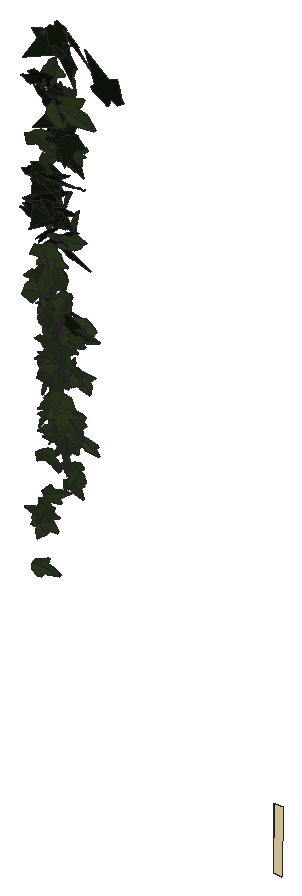
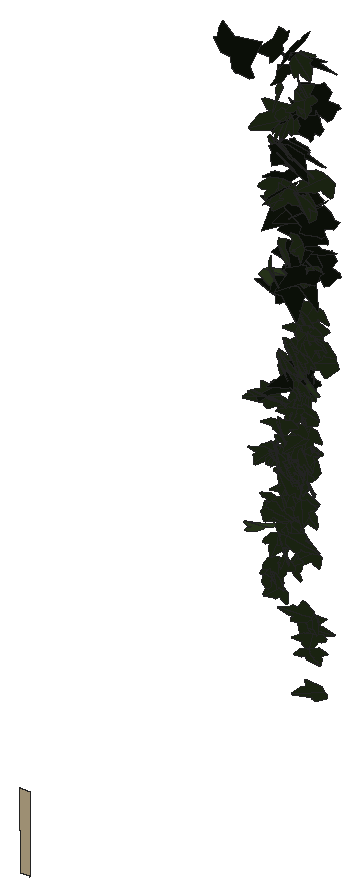
# SketchUp Ruby script. Lengths in inches.
U = 1.inch
M = Sketchup.active_model
def pt(a) = Geom::Point3d.new(a.map { |v| v * U })
def face(e, loops, mat)
  f = e.add_face(loops[0].map { |a| pt(a) })
  loops[1..].each { |l| e.add_face(l.map { |a| pt(a) }).erase! }
  f.material = f.back_material = mat if mat
  f
end
# faces: each face lists its corners as indices into pts; further lists are holes
def faces(e, pts, list, mat = nil) = list.each { |f| face(e, (f[0].is_a?(Array) ? f : [f]).map { |l| l.map { |i| pts[i] } }, mat) }
# xy, xz, yz: faces in a plane at the given z, y or x. An outline is a flat list of corners, or four numbers for a rectangle; further outlines are holes
def ring(l) = l.size == 4 ? [[l[0], l[1]], [l[2], l[1]], [l[2], l[3]], [l[0], l[3]]] : l.each_slice(2).to_a
def flat(e, list, mat, &to3) = list.each { |f| face(e, (f[0].is_a?(Array) ? f : [f]).map { |l| ring(l).map { |u, v| to3.(u, v) } }, mat) }
def xy(e, z, list, mat = nil) = flat(e, list, mat) { |x, y| [x, y, z] }
def xz(e, y, list, mat = nil) = flat(e, list, mat) { |x, z| [x, y, z] }
def yz(e, x, list, mat = nil) = flat(e, list, mat) { |y, z| [x, y, z] }
def lines(e, pts, list) = list.each { |a, b| e.add_line(pt(pts[a]), pt(pts[b])) }
# prism: a flat outline (further loops are holes) pulled along v
def prism(e, loops, v, mat = nil)
  f = face(e, loops, mat); d = Geom::Vector3d.new(v.map { |x| x * U })
  f.pushpull(f.normal.samedirection?(d) ? d.length : -d.length)
end
def box(e, o, s, mat = nil) = prism(e, [[o, [o[0] + s[0], o[1], o[2]], [o[0] + s[0], o[1] + s[1], o[2]], [o[0], o[1] + s[1], o[2]]]], [0, 0, s[2]], mat)
def at(x, y, z, deg = 0) = Geom::Transformation.translation(pt([x, y, z])) * Geom::Transformation.rotation(ORIGIN, Z_AXIS, deg.degrees)
def axes(o, x, y, z) = Geom::Transformation.new([*x, 0, *y, 0, *z, 0, *pt(o).to_a, 1])
def part(name) = M.definitions.add(name)
# library, detail: a bought-in or finely detailed component or shape, given as its bounding box
def library(name, o, s) = part(name).tap { |d| box(d.entities, o, s) }
def detail(e, o, s) = box(e.add_group.entities, o, s)
def put(e, d, t, mat = nil) = e.add_instance(d, t).tap { |i| i.material = mat if mat }
def group(e, t, mat = nil) = e.add_group.tap { |g| g.transformation = t; g.material = mat if mat }.entities
root = M.entities
M.materials.add("1026 AP 7946 SUNNY SIDE UP").color = [254, 231, 186]
M.materials.add("efeu1").color = [18, 25, 13]
M.materials.add("efeu2").color = [43, 57, 29]
c1 = part("ivyleaf_10")
p = [[0,0.5,-0.03],[-0.0625,2.02,-0.43],[-0.19,2.01,-0.46],[-0.54,1.05,-0.29],[-0.52,0.625,-0.18],[-0.83,0.76,-0.28],
  [-1.16,0.64,-0.33],[-1.15,0.33,-0.24],[-0.77,-0.39,0.02],[-0.3,-0.51,0.16],[0.04,-0.48,0.23],[-0.02,2.01,-0.4375],
  [-0.06,2.01,-0.43],[0.04,-0.49,0.23],[0.67,-0.49,0.14],[1.38,0.36,-0.2],[1.375,0.51,-0.24],[0.81,0.65,-0.19],
  [0.62,0.59,-0.15],[0.6,1.09,-0.28],[0.5,1.23,-0.31]]
faces(c1.entities,p,[[0,1,2,3,4,5,6,7,8,9,10],[11,12,0,13,14,15,16,17,18,19,20]],"efeu2")
c2 = part("ivyleaf_9")
p = [[1.54,2.16,1.25],[1.36,2.04,1.19],[-0.21,0.99,0.68],[-0.71,1.11,0.82],[-0.85,0.86,0.67],[-0.8,0.17,0.21],
  [-0.9,-0.01,0.1],[-0.67,-0.16,-0.02],[-0.08,-0.08,-0.05],[-0.03,-0.6,-0.4],[0.65,-0.88,-0.66],[0.83,-0.6,-0.49],
  [1.29,-0.42,-0.43],[1.8125,-0.07,-0.26],[1.21,0.44,0.15]]
faces(c2.entities,p,[[0,1,2,3,4,5,6,7,8,9,10,11,12,13,14]],"efeu1")
xz(root,213.099,[[153.231,245.999,153.241,247.999,152.988,248,152.981,246]],"1026 AP 7946 SUNNY SIDE UP")
p = [[152.981,213.099,246],[152.988,213.099,248],[152.981,213.1,248],[152.978,213.099,246]]
faces(root,p,[[0,1,2,3]],"1026 AP 7946 SUNNY SIDE UP")
put(root,c1,axes([145.59,212.75,264.89],[-0.28973,-0.04705,-0.17397],[0.26689,0.0118,-0.19442],[0.06726,-0.24948,0.0221]),"1026 AP 7946 SUNNY SIDE UP")
put(root,c2,axes([145.47,212.61,262.8],[0.36964,-0.02084,0.11456],[0.16957,-0.03713,-0.242],[0.05438,0.25744,-0.02409]),"1026 AP 7946 SUNNY SIDE UP")
put(root,c1,axes([146.01,212.67,254.15],[0.01993,-0.00468,-0.21341],[-0.32565,0.00536,-0.01315],[0.00886,0.20745,-0.00326]),"1026 AP 7946 SUNNY SIDE UP")
put(root,c1,axes([145.77,212.74,260.93],[-0.36692,-0.08893,-0.03495],[0.07197,-0.02757,-0.25381],[0.1309,-0.23411,0.04158]),"1026 AP 7946 SUNNY SIDE UP")
put(root,c1,axes([145.84,212.76,260.0625],[-0.22002,0.18793,0.06334],[-0.10512,0.02457,-0.23808],[-0.29205,-0.15042,0.03797]),"1026 AP 7946 SUNNY SIDE UP")
put(root,c1,axes([145.82,213.1875,267.8],[-0.05734,-0.22404,0.10374],[-0.00507,-0.10264,-0.23411],[0.38702,-0.03454,0.0123]),"1026 AP 7946 SUNNY SIDE UP")
put(root,c1,axes([145.82,212.67,261.2],[-0.02168,-0.25461,-0.00797],[-0.00088,0.00633,-0.26264],[0.40047,-0.01377,-0.00101]),"1026 AP 7946 SUNNY SIDE UP")
put(root,c1,axes([145.54,212.5625,260.49],[-0.05462,-0.05264,-0.23677],[0.34552,0.07617,-0.05181],[0.13313,-0.21929,0.03733]),"1026 AP 7946 SUNNY SIDE UP")
put(root,c1,axes([145.8,212.92,258.95],[-0.32874,0.02394,-0.0091],[0.01137,-0.01548,-0.21636],[-0.03855,-0.20869,0.01377]),"1026 AP 7946 SUNNY SIDE UP")
put(root,c1,axes([145.55,213.07,259.4375],[0.00437,-0.01694,-0.21177],[0.28532,-0.09735,0.01023],[-0.15389,-0.18097,0.01295]),"1026 AP 7946 SUNNY SIDE UP")
put(root,c1,axes([145.84,212.98,258.43],[-0.04466,-0.19756,0.04918],[-0.01328,-0.04815,-0.20589],[0.31972,-0.02959,-0.00168]),"1026 AP 7946 SUNNY SIDE UP")
put(root,c1,axes([145.8,212.84,253.71],[0.27005,0.08927,-0.06744],[-0.07271,-0.05294,-0.19813],[-0.15866,0.17619,-0.02398]),"1026 AP 7946 SUNNY SIDE UP")
put(root,c1,axes([145.77,212.99,257.84],[0.21885,-0.15832,0.05318],[0.03274,-0.05137,-0.2167],[0.26024,0.13961,-0.01746]),"1026 AP 7946 SUNNY SIDE UP")
put(root,c1,axes([145.8125,213.09,257.24],[-0.06075,-0.20631,-0.01788],[0.03651,0.01204,-0.21512],[0.32334,-0.04012,0.02093]),"1026 AP 7946 SUNNY SIDE UP")
put(root,c1,axes([145.82,213.05,257.68],[-0.18649,0.16259,0.04429],[0.05147,-0.02813,0.20693],[0.25901,0.12266,-0.00924]),"1026 AP 7946 SUNNY SIDE UP")
put(root,c1,axes([146.04,213.08,256.36],[-0.10447,-0.0008,0.20049],[-0.27494,-0.09005,-0.0624],[0.13437,-0.18488,0.02819]),"1026 AP 7946 SUNNY SIDE UP")
put(root,c1,axes([145.79,213.24,261.26],[-0.03188,0.03985,-0.2062],[-0.02068,-0.20121,-0.04103],[-0.32059,0.00902,0.02315]),"1026 AP 7946 SUNNY SIDE UP")
put(root,c1,axes([145.85,212.97,258.5],[-0.1948,-0.16449,0.00997],[0.00967,-0.01788,-0.21163],[0.259,-0.12305,0.0154]),"1026 AP 7946 SUNNY SIDE UP")
put(root,c2,axes([145.58,212.58,266.6875],[0.37695,0.05787,0.09665],[0.15159,-0.00285,-0.2529],[-0.0831,0.2573,-0.02295]),"1026 AP 7946 SUNNY SIDE UP")
put(root,c1,axes([145.67,212.86,259.91],[0.1097,-0.17416,-0.087],[0.14964,-0.04622,0.18104],[-0.26425,-0.09847,0.0664]),"1026 AP 7946 SUNNY SIDE UP")
put(root,c1,axes([145.77,212.87,257.9],[-0.09767,-0.16191,0.13668],[0.05553,0.12927,0.17907],[-0.32536,0.07067,-0.01047]),"1026 AP 7946 SUNNY SIDE UP")
put(root,c1,axes([145.82,213.02,266.74],[0.15259,0.21371,-0.05953],[-0.02659,-0.05708,-0.24199],[-0.34759,0.09819,-0.00762]),"1026 AP 7946 SUNNY SIDE UP")
put(root,c1,axes([145.91,212.84,256.95],[-0.01576,-0.18278,0.09988],[-0.008,-0.09786,-0.18915],[0.326,-0.01124,0.00019]),"1026 AP 7946 SUNNY SIDE UP")
put(root,c1,axes([145.95,212.77,259.83],[-0.30808,0.12702,0.05819],[-0.09849,0.00511,-0.23866],[-0.19462,-0.20365,0.02866]),"1026 AP 7946 SUNNY SIDE UP")
put(root,c1,axes([145.81,212.93,262.74],[0.21868,0.1892,-0.00643],[0.00969,-0.01359,-0.24161],[-0.29756,0.1386,-0.01259]),"1026 AP 7946 SUNNY SIDE UP")
put(root,c1,axes([145.81,212.76,254.02],[0.23662,0.15145,0.01035],[0.02711,-0.00421,-0.21941],[-0.23703,0.1507,-0.01476]),"1026 AP 7946 SUNNY SIDE UP")
put(root,c1,axes([145.86,212.95,261.02],[0.32692,0.07435,-0.02185],[-0.02057,-0.02736,-0.22657],[-0.12001,0.20723,-0.02068]),"1026 AP 7946 SUNNY SIDE UP")
put(root,c2,axes([146.1,212.9375,267.71],[-0.41241,-0.06339,0.06128],[-0.07307,-0.05888,-0.27439],[0.11598,-0.2625,0.04504]),"1026 AP 7946 SUNNY SIDE UP")
put(root,c2,axes([145.75,212.78,263.45],[0.08478,-0.25861,-0.00597],[-0.01338,0.00265,-0.27201],[0.40647,0.05403,-0.00771]),"1026 AP 7946 SUNNY SIDE UP")
put(root,c1,axes([146.06,212.875,258.52],[-0.31127,-0.01563,0.10276],[-0.14527,-0.06098,-0.19891],[0.06438,-0.21316,0.04801]),"1026 AP 7946 SUNNY SIDE UP")
put(root,c1,axes([145.9,213.05,264.47],[0.33964,-0.09587,-0.00442],[-0.018,-0.01659,-0.2427],[0.14979,0.2154,-0.01914]),"1026 AP 7946 SUNNY SIDE UP")
put(root,c2,axes([145.61,212.69,263.73],[0.05713,-0.03664,0.25131],[0.37481,-0.05905,-0.04602],[0.10108,0.23967,0.0286]),"1026 AP 7946 SUNNY SIDE UP")
put(root,c1,axes([145.95,213.125,260.87],[0.24903,-0.13479,-0.03773],[-0.05968,0.01056,-0.21353],[0.21103,0.16204,-0.01586]),"1026 AP 7946 SUNNY SIDE UP")
put(root,c1,axes([146,212.66,254.26],[-0.12119,-0.18463,0.09215],[-0.03974,-0.08741,-0.20639],[0.32086,-0.08056,0.00924]),"1026 AP 7946 SUNNY SIDE UP")
put(root,c1,axes([145.97,212.94,266.82],[0.02822,-0.21527,0.14551],[0.0118,-0.14232,-0.22334],[0.40574,0.01911,-0.00363]),"1026 AP 7946 SUNNY SIDE UP")
put(root,c2,axes([146,212.74,263.08],[-0.31724,-0.16191,0.00747],[0.01037,-0.02123,-0.26577],[0.2547,-0.2008,0.02013]),"1026 AP 7946 SUNNY SIDE UP")
put(root,c1,axes([145.75,212.81,264.16],[-0.02777,0.0172,-0.24949],[0.20138,-0.20575,-0.02587],[-0.32451,-0.12915,0.0053]),"1026 AP 7946 SUNNY SIDE UP")
put(root,c1,axes([145.87,212.69,254.4],[-0.24154,0.09852,-0.11823],[0.09896,-0.10794,-0.18198],[-0.21699,-0.15889,0.04861]),"1026 AP 7946 SUNNY SIDE UP")
put(root,c1,axes([145.9375,212.93,261.67],[0.27575,-0.13634,0.01659],[0.00434,-0.02387,-0.2283],[0.21597,0.17456,-0.01659]),"1026 AP 7946 SUNNY SIDE UP")
put(root,c2,axes([145.81,212.97,262.74],[0.0242,-0.11537,-0.22412],[0.04115,0.21685,-0.11565],[0.38409,-0.01596,0.02651]),"1026 AP 7946 SUNNY SIDE UP")
put(root,c1,axes([145.86,213.12,263.42],[-0.20136,0.12932,-0.13801],[0.11487,-0.11562,-0.18658],[-0.27021,-0.14552,0.02353]),"1026 AP 7946 SUNNY SIDE UP")
put(root,c1,axes([145.93,212.96,260.71],[0.31644,-0.0875,0.02252],[0.01942,-0.02742,-0.22528],[0.14067,0.20062,-0.01955]),"1026 AP 7946 SUNNY SIDE UP")
put(root,c1,axes([145.9,212.69,261.71],[-0.37438,-0.02438,-0.08866],[0.13751,-0.11334,-0.21718],[-0.02852,-0.22633,0.11664]),"1026 AP 7946 SUNNY SIDE UP")
put(root,c1,axes([145.88,212.68,260.93],[0.37868,-0.05962,0.04455],[0.06919,-0.00356,-0.25551],[0.09327,0.24471,0.00866]),"1026 AP 7946 SUNNY SIDE UP")
put(root,c1,axes([145.98,212.99,260.48],[0.10806,-0.19248,0.06351],[0.02407,-0.06113,-0.21082],[0.31742,0.07016,-0.00563]),"1026 AP 7946 SUNNY SIDE UP")
put(root,c1,axes([146.02,213,257.92],[0.18116,-0.17105,-0.06316],[-0.041,0.05512,-0.21195],[0.28224,0.1178,0.00975]),"1026 AP 7946 SUNNY SIDE UP")
put(root,c1,axes([145.92,212.92,261.33],[0.32179,0.08564,0.00194],[0.0141,-0.01782,-0.22773],[-0.13393,0.20388,-0.01931]),"1026 AP 7946 SUNNY SIDE UP")
put(root,c2,axes([145.75,212.82,266.01],[0.02937,-0.02475,0.25452],[0.1948,-0.21395,-0.03296],[0.33861,0.12523,-0.00311]),"1026 AP 7946 SUNNY SIDE UP")
put(root,c1,axes([146.04,212.89,258.61],[-0.32998,0.08353,0.01615],[-0.03258,-0.01107,-0.23202],[-0.12947,-0.21011,0.01722]),"1026 AP 7946 SUNNY SIDE UP")
put(root,c1,axes([146.03,213.0625,259.77],[-0.17952,0.17257,0.05563],[-0.06183,0.03745,-0.2126],[-0.27705,-0.12018,0.0114]),"1026 AP 7946 SUNNY SIDE UP")
put(root,c1,axes([145.76,212.94,259.27],[-0.07183,0.0185,0.20502],[0.31252,0.02479,0.04479],[-0.03168,0.20258,-0.023]),"1026 AP 7946 SUNNY SIDE UP")
put(root,c1,axes([146,212.6,260.17],[0.0902,0.02622,-0.24489],[0.04899,0.2417,0.0366],[0.37308,-0.03808,0.0544]),"1026 AP 7946 SUNNY SIDE UP")
put(root,c1,axes([146,212.87,259.58],[0.05077,0.23135,0.04639],[-0.03961,0.04727,-0.23825],[-0.36809,0.02683,0.03204]),"1026 AP 7946 SUNNY SIDE UP")
put(root,c1,axes([146.05,212.9,259.35],[0.1868,-0.20286,-0.01011],[-0.02446,0.00092,-0.24181],[0.31834,0.11911,-0.01264]),"1026 AP 7946 SUNNY SIDE UP")
put(root,c1,axes([145.81,212.55,252.62],[0.07754,0.05786,0.2],[0.24428,0.1169,-0.076],[-0.20365,0.16226,-0.01501]),"1026 AP 7946 SUNNY SIDE UP")
put(root,c1,axes([146.07,212.83,257.22],[-0.20313,-0.17743,-0.00341],[0.0212,-0.00697,-0.22562],[0.27822,-0.12902,0.0147]),"1026 AP 7946 SUNNY SIDE UP")
put(root,c1,axes([145.8,212.8,258.34],[0.12887,-0.04596,-0.20126],[0.3148,0.00861,0.0846],[-0.01519,-0.21144,0.0459]),"1026 AP 7946 SUNNY SIDE UP")
put(root,c1,axes([145.97,213.07,259.42],[0.24017,0.14425,0.0353],[0.05054,0.01461,-0.21603],[-0.22729,0.15567,-0.01074]),"1026 AP 7946 SUNNY SIDE UP")
put(root,c2,axes([146.2,212.6,262.45],[-0.05921,0.24846,-0.0727],[0.01497,-0.07136,-0.25929],[-0.40646,-0.03882,0.00104]),"1026 AP 7946 SUNNY SIDE UP")
put(root,c1,axes([145.92,213,258.71],[0.1663,0.13703,0.12335],[0.13005,0.08615,-0.17749],[-0.25396,0.13384,-0.01012]),"1026 AP 7946 SUNNY SIDE UP")
put(root,c2,axes([146.3,213.02,265.61],[-0.3979,0.01273,0.04292],[-0.06716,-0.02634,-0.25957],[-0.01292,-0.25509,0.02744]),"1026 AP 7946 SUNNY SIDE UP")
put(root,c1,axes([146.09,212.69,257.92],[0.09742,-0.15066,-0.16725],[0.01381,0.16928,-0.15823],[0.34701,0.03556,0.05325]),"1026 AP 7946 SUNNY SIDE UP")
put(root,c1,axes([145.95,213.03,260.08],[0.282,-0.06227,0.11212],[0.15006,-0.05636,-0.19493],[0.12863,0.20226,-0.01841]),"1026 AP 7946 SUNNY SIDE UP")
put(root,c1,axes([145.92,212.87,254.55],[-0.07451,-0.04142,0.20063],[0.19035,0.15325,0.06474],[-0.24902,0.12954,-0.01055]),"1026 AP 7946 SUNNY SIDE UP")
put(root,c2,axes([145.91,212.69,264.0625],[0.04715,-0.26395,-0.03636],[0.0542,0.03757,-0.27061],[0.4149,0.02509,0.03948]),"1026 AP 7946 SUNNY SIDE UP")
put(root,c1,axes([145.94,212.63,255.875],[-0.22369,-0.03186,-0.145],[0.22513,-0.00853,-0.14733],[0.02605,-0.19981,0.02821]),"1026 AP 7946 SUNNY SIDE UP")
put(root,c2,axes([146.21,213.08,265.58],[0.00107,0.19395,-0.17631],[0.00221,-0.17225,-0.20081],[-0.40786,-0.00043,-0.00155]),"1026 AP 7946 SUNNY SIDE UP")
put(root,c1,axes([145.92,213.12,259.99],[0.07796,-0.05244,0.19581],[0.24756,-0.10797,-0.07351],[0.18739,0.16444,0.01565]),"1026 AP 7946 SUNNY SIDE UP")
put(root,c2,axes([146.14,212.52,263.47],[0.17587,0.24584,-0.01816],[-0.01353,-0.01699,-0.27834],[-0.38748,0.11217,0.00147]),"1026 AP 7946 SUNNY SIDE UP")
put(root,c1,axes([146.06,212.95,257.83],[0.20586,-0.15143,0.0668],[0.05691,-0.05548,-0.20637],[0.25324,0.13557,-0.00793]),"1026 AP 7946 SUNNY SIDE UP")
put(root,c2,axes([146.29,212.68,262.92],[-0.37193,0.09082,-0.04667],[0.04453,-0.05259,-0.25833],[-0.15363,-0.23512,0.0381]),"1026 AP 7946 SUNNY SIDE UP")
put(root,c1,axes([146.26,212.77,255.52],[-0.15104,0.10911,-0.1567],[-0.12867,0.13005,0.1495],[0.26561,0.12505,-0.01669]),"1026 AP 7946 SUNNY SIDE UP")
put(root,c1,axes([146.375,212.74,256.41],[-0.11978,0.03781,0.20691],[-0.32093,-0.0089,-0.07816],[-0.0078,-0.21442,0.03844]),"1026 AP 7946 SUNNY SIDE UP")
put(root,c2,axes([145.89,212.77,260.13],[0.34112,0.03891,0.10585],[0.15709,0.02361,-0.22686],[-0.07112,0.23878,0.00662]),"1026 AP 7946 SUNNY SIDE UP")
put(root,c2,axes([145.91,212.46,263.97],[0.39777,0.05556,0.09586],[0.1239,0.06679,-0.26228],[-0.11637,0.26102,0.0484]),"1026 AP 7946 SUNNY SIDE UP")
put(root,c2,axes([146.12,212.6875,262.95],[0.29532,0.16723,-0.05175],[-0.04694,-0.04336,-0.25901],[-0.27096,0.18978,-0.01154]),"1026 AP 7946 SUNNY SIDE UP")
put(root,c1,axes([146,212.9,267.05],[0.23895,-0.12864,0.17362],[0.19057,-0.11852,-0.20559],[0.27466,0.19415,-0.00841]),"1026 AP 7946 SUNNY SIDE UP")
put(root,c1,axes([146.24,213.02,260.89],[0.21959,-0.14353,-0.1322],[-0.11361,0.10679,-0.20474],[0.27969,0.15606,0.02063]),"1026 AP 7946 SUNNY SIDE UP")
put(root,c2,axes([146.05,212.92,268.04],[0.15608,-0.2195,-0.14572],[-0.12021,0.11888,-0.24679],[0.3915,0.12401,-0.01768]),"1026 AP 7946 SUNNY SIDE UP")
put(root,c2,axes([146.39,213.09,265.57],[-0.33075,0.14047,0.00235],[-0.02246,-0.01874,-0.25956],[-0.21975,-0.20952,0.023]),"1026 AP 7946 SUNNY SIDE UP")
put(root,c1,axes([146.21,212.71,260.02],[0.09239,-0.22755,0.06493],[0.01909,-0.06328,-0.24245],[0.37133,0.05987,-0.00369]),"1026 AP 7946 SUNNY SIDE UP")
put(root,c1,axes([146.2,212.74,258.02],[-0.3385,0.02485,-0.03016],[0.04141,-0.02686,-0.2221],[-0.04418,-0.21561,0.02289]),"1026 AP 7946 SUNNY SIDE UP")
put(root,c1,axes([146.35,212.99,257.13],[-0.2408,-0.0835,0.12537],[-0.12556,-0.1014,-0.1751],[0.1959,-0.16762,0.04189]),"1026 AP 7946 SUNNY SIDE UP")
put(root,c1,axes([146.27,212.63,256.6],[0.08314,-0.19354,-0.09959],[-0.05242,0.08989,-0.20601],[0.33533,0.06204,-0.00751]),"1026 AP 7946 SUNNY SIDE UP")
put(root,c1,axes([146.21,212.79,259.24],[-0.19753,0.20055,0.00014],[-0.01803,-0.00836,-0.2434],[-0.31484,-0.12535,0.01385]),"1026 AP 7946 SUNNY SIDE UP")
put(root,c1,axes([146.22,213.09,266.26],[-0.30501,0.16894,-0.0124],[-0.00606,-0.02415,-0.26427],[-0.26635,-0.19291,0.02022]),"1026 AP 7946 SUNNY SIDE UP")
put(root,c1,axes([146.21,212.77,259.49],[-0.15841,0.21701,0.01103],[-0.01324,0.00653,-0.24639],[-0.34129,-0.10098,0.00444]),"1026 AP 7946 SUNNY SIDE UP")
put(root,c2,axes([146.33,212.83,262.2],[0.05287,0.24522,-0.03991],[-0.01658,-0.03905,-0.25517],[-0.39037,0.03487,0.00543]),"1026 AP 7946 SUNNY SIDE UP")
put(root,c1,axes([146.07,212.68,261.17],[0.2909,-0.06203,0.15734],[0.22254,-0.05895,-0.20117],[0.13388,0.23277,-0.00747]),"1026 AP 7946 SUNNY SIDE UP")
put(root,c1,axes([146.26,213.04,258.0625],[0.33077,-0.04389,-0.01085],[-0.02203,-0.01702,-0.22056],[0.06737,0.20992,-0.01887]),"1026 AP 7946 SUNNY SIDE UP")
put(root,c2,axes([146.21,213.04,266.22],[-0.04481,-0.25881,0.04694],[-0.01002,-0.04662,-0.2685],[0.41349,-0.02918,-0.00142]),"1026 AP 7946 SUNNY SIDE UP")
put(root,c1,axes([146.41,212.59,258.61],[0.10281,-0.06691,-0.23017],[-0.09168,0.21959,-0.08418],[0.3545,0.07619,0.04498]),"1026 AP 7946 SUNNY SIDE UP")
put(root,c1,axes([146.28,212.98,258.51],[-0.28781,0.07368,-0.09907],[0.06895,-0.12282,-0.18284],[-0.17814,-0.16658,0.08929]),"1026 AP 7946 SUNNY SIDE UP")
put(root,c2,axes([146.45,213.09,265.41],[-0.35341,0.07612,-0.10335],[0.12398,-0.07607,-0.24085],[-0.15509,-0.23426,0.04297]),"1026 AP 7946 SUNNY SIDE UP")
put(root,c1,axes([146.32,213.13,263.19],[0.15441,-0.20431,0.07674],[0.04149,-0.07121,-0.23384],[0.34005,0.10146,-0.00631]),"1026 AP 7946 SUNNY SIDE UP")
put(root,c1,axes([146.39,212.83,257.19],[-0.01234,-0.20926,0.02063],[-0.00018,-0.02123,-0.21585],[0.33073,-0.00782,0.00065]),"1026 AP 7946 SUNNY SIDE UP")
put(root,c2,axes([146.31,213.07,264.94],[-0.18365,-0.21999,-0.04115],[0.06565,0.02139,-0.25501],[0.34503,-0.12117,0.02662]),"1026 AP 7946 SUNNY SIDE UP")
put(root,c1,axes([146.37,213.12,258.95],[0.14832,-0.19052,0.04642],[0.03373,-0.04087,-0.21925],[0.30639,0.09673,0.00166]),"1026 AP 7946 SUNNY SIDE UP")
put(root,c1,axes([146.35,213.08,266.15],[-0.09147,0.24594,0.01201],[-0.00349,0.01002,-0.2603],[-0.38704,-0.05822,-0.00049]),"1026 AP 7946 SUNNY SIDE UP")
put(root,c1,axes([146.34,213.13,259.06],[0.3119,0.09167,-0.00803],[0.00347,-0.02447,-0.22399],[-0.14469,0.19702,-0.02267]),"1026 AP 7946 SUNNY SIDE UP")
put(root,c1,axes([146.43,212.8125,256.36],[0.0676,0.1858,-0.12255],[-0.10584,-0.10547,-0.19368],[-0.33131,0.0716,0.03686]),"1026 AP 7946 SUNNY SIDE UP")
put(root,c2,axes([146.22,213.08,267.3],[0.03968,-0.22841,0.13614],[0.05571,-0.12992,-0.23676],[0.41221,0.03954,0.01889]),"1026 AP 7946 SUNNY SIDE UP")
put(root,c1,axes([146.44,212.78,260.31],[-0.14663,-0.16583,0.1394],[0.01875,-0.15234,-0.18348],[0.33696,-0.06368,0.07087]),"1026 AP 7946 SUNNY SIDE UP")
put(root,c1,axes([146.45,212.97,256.09],[0.13056,-0.18267,-0.04844],[-0.04333,0.03794,-0.20628],[0.29301,0.087,-0.00892]),"1026 AP 7946 SUNNY SIDE UP")
put(root,c2,axes([146.25,213.11,264.61],[0.10031,-0.22844,-0.09142],[0.00184,0.09065,-0.24256],[0.38461,0.05915,0.02501]),"1026 AP 7946 SUNNY SIDE UP")
put(root,c1,axes([146.39,212.9,255.87],[-0.07221,0.20258,0.0026],[-0.00603,0.00054,-0.21395],[-0.31848,-0.04594,0.00346]),"1026 AP 7946 SUNNY SIDE UP")
put(root,c1,axes([146.39,212.92,260.41],[0.28806,-0.14167,0.03114],[0.01499,-0.03813,-0.2375],[0.22756,0.18185,-0.02378]),"1026 AP 7946 SUNNY SIDE UP")
put(root,c1,axes([146.29,213.07,264.5],[0.3481,0.06465,0.10209],[0.12119,0.07974,-0.23136],[-0.14053,0.22891,0.05336]),"1026 AP 7946 SUNNY SIDE UP")
put(root,c1,axes([146.59,213.15,256.94],[0.12069,0.09855,-0.1648],[-0.23655,-0.07225,-0.12022],[-0.17825,0.16261,0.04796]),"1026 AP 7946 SUNNY SIDE UP")
put(root,c1,axes([146.33,212.86,257.25],[-0.27796,0.02353,0.12965],[0.19629,-0.01488,0.18362],[0.04373,0.2164,-0.00018]),"1026 AP 7946 SUNNY SIDE UP")
put(root,c1,axes([146.39,213.11,264.65],[-0.31362,-0.13231,-0.0825],[0.1498,-0.00364,-0.24051],[0.1908,-0.21462,0.05321]),"1026 AP 7946 SUNNY SIDE UP")
put(root,c1,axes([146.43,213.07,266.8125],[-0.15482,0.23717,-0.01422],[-0.00276,-0.01712,-0.26451],[-0.37367,-0.09814,0.00784]),"1026 AP 7946 SUNNY SIDE UP")
put(root,c1,axes([146.42,213.12,265.58],[0.33969,-0.12064,0.02454],[0.0251,-0.02163,-0.25478],[0.19194,0.21634,-0.01012]),"1026 AP 7946 SUNNY SIDE UP")
put(root,c1,axes([146.48,212.84,256.27],[-0.03089,-0.22177,-0.01228],[0.03701,0.00856,-0.22812],[0.34715,-0.02064,0.02323]),"1026 AP 7946 SUNNY SIDE UP")
put(root,c1,axes([146.33,212.85,258.23],[0.17117,-0.11483,0.16696],[0.18788,-0.1107,-0.16348],[0.25053,0.16148,0.00852]),"1026 AP 7946 SUNNY SIDE UP")
put(root,c1,axes([146.5,213.1,258.4],[0.11303,-0.20193,-0.05557],[-0.00492,0.05479,-0.21996],[0.32816,0.07038,0.01584]),"1026 AP 7946 SUNNY SIDE UP")
put(root,c1,axes([146.47,212.625,257.64],[0.3745,0.01007,-0.0401],[-0.05997,-0.01855,-0.24509],[-0.0203,0.24063,-0.0158]),"1026 AP 7946 SUNNY SIDE UP")
put(root,c1,axes([146.48,212.95,256.56],[-0.01735,-0.08756,0.18792],[0.05264,-0.18146,-0.08847],[0.31449,0.02554,0.02518]),"1026 AP 7946 SUNNY SIDE UP")
put(root,c1,axes([146.46,213.04,256.23],[-0.23033,-0.13092,-0.06107],[0.09356,0.02065,-0.20085],[0.20517,-0.15639,0.02303]),"1026 AP 7946 SUNNY SIDE UP")
put(root,c1,axes([146.53,213.08,258.18],[0.30998,-0.08479,-0.0498],[-0.07607,0.00848,-0.22074],[0.13286,0.20269,-0.0102]),"1026 AP 7946 SUNNY SIDE UP")
put(root,c1,axes([146.55,212.95,255.6],[-0.25024,-0.13581,-0.01316],[0.02975,-0.00373,-0.21499],[0.2123,-0.15955,0.01462]),"1026 AP 7946 SUNNY SIDE UP")
put(root,c1,axes([146.51,213.03,258.31],[-0.30356,0.0795,-0.04118],[0.04741,-0.03254,-0.21445],[-0.13197,-0.19454,0.01768]),"1026 AP 7946 SUNNY SIDE UP")
put(root,c1,axes([146.87,212.7,262.21],[-0.00595,0.29114,-0.00133],[-0.44032,-0.00283,0.08213],[0.12532,0.00387,0.28851]),"1026 AP 7946 SUNNY SIDE UP")
put(root,c1,axes([146.55,212.88,260.375],[0.14543,-0.22461,0.01395],[-0.00344,-0.01691,-0.25019],[0.35393,0.09213,-0.00816]),"1026 AP 7946 SUNNY SIDE UP")
put(root,c1,axes([146.47,212.61,257.26],[0.26747,0.16814,-0.00693],[0.00974,-0.01717,-0.24591],[-0.26447,0.16941,-0.01607]),"1026 AP 7946 SUNNY SIDE UP")
put(root,c2,axes([146.4375,212.56,263.89],[0.40408,0.10381,0.01431],[-0.04375,0.10175,-0.26379],[-0.15864,0.23635,0.10919]),"1026 AP 7946 SUNNY SIDE UP")
put(root,c1,axes([146.51,213.03,258.29],[-0.30848,0.03059,-0.07773],[0.10741,-0.04606,-0.20203],[-0.07012,-0.20515,0.03248]),"1026 AP 7946 SUNNY SIDE UP")
put(root,c1,axes([146.48,213.25,262.63],[0.17759,-0.13005,0.16419],[0.15488,-0.12638,-0.17807],[0.28498,0.14973,-0.00554]),"1026 AP 7946 SUNNY SIDE UP")
put(root,c1,axes([146.34,212.75,259.16],[-0.02886,-0.01791,-0.24462],[0.31203,-0.1326,-0.00627],[-0.20667,-0.1977,0.02468]),"1026 AP 7946 SUNNY SIDE UP")
put(root,c1,axes([146.61,213.06,255.3],[-0.29241,0.06534,-0.051],[0.02382,-0.094,-0.18562],[-0.12704,-0.16802,0.08258]),"1026 AP 7946 SUNNY SIDE UP")
put(root,c2,axes([146.88,212.83,259.58],[-0.06209,0.25707,-0.01903],[-0.40211,-0.03647,0.03709],[0.05174,0.02502,0.26547]),"1026 AP 7946 SUNNY SIDE UP")
put(root,c1,axes([146.82,213.19,259.58],[-0.34233,0.10731,0.099],[-0.21323,-0.21072,-0.0758],[0.07449,-0.11006,0.23803]),"1026 AP 7946 SUNNY SIDE UP")
put(root,c1,axes([146.49,213.03,255.04],[-0.25096,0.00812,-0.13104],[0.18518,-0.06876,-0.15709],[-0.07685,-0.19219,0.04939]),"1026 AP 7946 SUNNY SIDE UP")
put(root,c1,axes([146.69,213.07,255.28],[-0.07365,-0.11696,0.16347],[-0.00025,-0.16374,-0.12482],[0.31081,-0.02785,0.03864]),"1026 AP 7946 SUNNY SIDE UP")
put(root,c2,axes([146.4375,213.02,267.89],[0.2563,-0.20314,0.04841],[0.02035,-0.05113,-0.2677],[0.32764,0.16209,-0.02124]),"1026 AP 7946 SUNNY SIDE UP")
put(root,c1,axes([146.5,212.8,256.71],[0.24642,0.04837,0.16329],[0.24362,0.03359,-0.16847],[-0.09131,0.22016,-0.00879]),"1026 AP 7946 SUNNY SIDE UP")
put(root,c2,axes([146.46,212.71,261.99],[0.25003,-0.13845,0.15679],[0.16216,-0.11395,-0.21734],[0.281,0.18895,-0.01408]),"1026 AP 7946 SUNNY SIDE UP")
put(root,c1,axes([146.67,212.86,256.95],[-0.27918,0.04071,-0.13947],[0.16947,-0.1022,-0.17757],[-0.14438,-0.19867,0.06125]),"1026 AP 7946 SUNNY SIDE UP")
put(root,c1,axes([146.45,212.64,266.01],[0.23601,0.14268,0.3195],[0.37275,0.199,-0.2119],[-0.38466,0.28038,-0.00931]),"1026 AP 7946 SUNNY SIDE UP")
put(root,c1,axes([146.74,213.02,258.16],[0.22432,0.11864,0.10922],[0.14531,0.05302,-0.19014],[-0.20279,0.16923,-0.01543]),"1026 AP 7946 SUNNY SIDE UP")
put(root,c1,axes([146.74,212.88,259.43],[0.09122,-0.00955,0.2258],[0.24896,0.15883,-0.0351],[-0.23891,0.16187,0.04963]),"1026 AP 7946 SUNNY SIDE UP")
put(root,c1,axes([146.89,213.04,256.36],[-0.13841,-0.19864,0.02343],[0.31003,-0.09056,-0.02779],[0.05336,0.01088,0.22223]),"1026 AP 7946 SUNNY SIDE UP")
put(root,c2,axes([148.03,212.64,266.91],[0.10967,-0.0895,0.36989],[-0.26971,0.31651,0.11729],[-0.51643,-0.18431,0.0173]),"1026 AP 7946 SUNNY SIDE UP")
